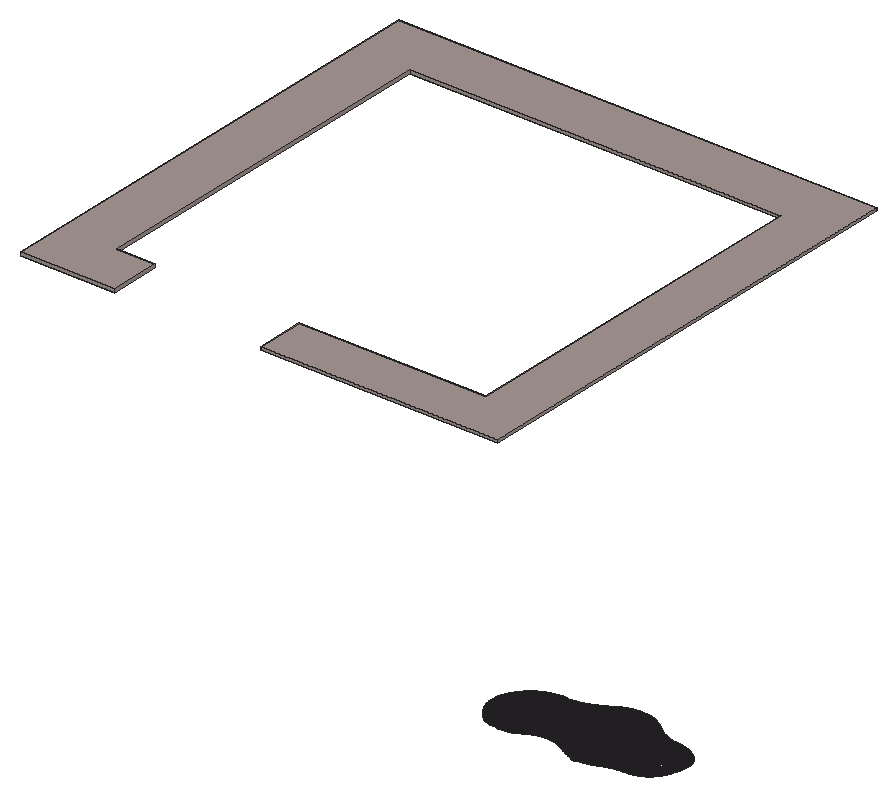
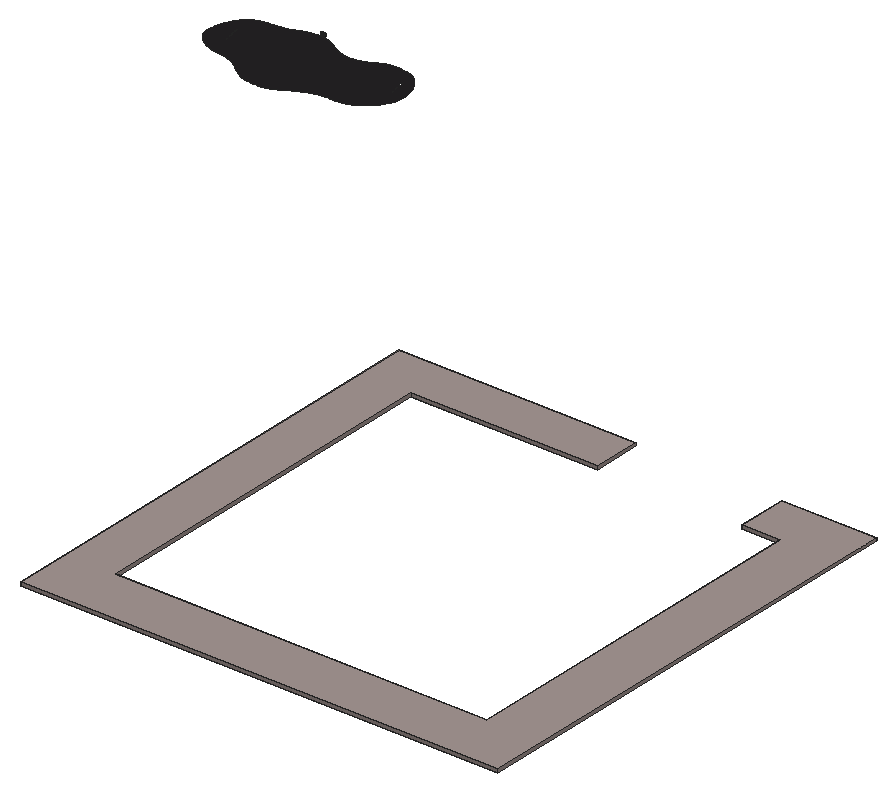
# SketchUp Ruby script. Lengths in inches.
U = 1.inch
M = Sketchup.active_model
def pt(a) = Geom::Point3d.new(a.map { |v| v * U })
def face(e, loops, mat)
  f = e.add_face(loops[0].map { |a| pt(a) })
  loops[1..].each { |l| e.add_face(l.map { |a| pt(a) }).erase! }
  f.material = f.back_material = mat if mat
  f
end
# faces: each face lists its corners as indices into pts; further lists are holes
def faces(e, pts, list, mat = nil) = list.each { |f| face(e, (f[0].is_a?(Array) ? f : [f]).map { |l| l.map { |i| pts[i] } }, mat) }
# xy, xz, yz: faces in a plane at the given z, y or x. An outline is a flat list of corners, or four numbers for a rectangle; further outlines are holes
def ring(l) = l.size == 4 ? [[l[0], l[1]], [l[2], l[1]], [l[2], l[3]], [l[0], l[3]]] : l.each_slice(2).to_a
def flat(e, list, mat, &to3) = list.each { |f| face(e, (f[0].is_a?(Array) ? f : [f]).map { |l| ring(l).map { |u, v| to3.(u, v) } }, mat) }
def xy(e, z, list, mat = nil) = flat(e, list, mat) { |x, y| [x, y, z] }
def xz(e, y, list, mat = nil) = flat(e, list, mat) { |x, z| [x, y, z] }
def yz(e, x, list, mat = nil) = flat(e, list, mat) { |y, z| [x, y, z] }
def lines(e, pts, list) = list.each { |a, b| e.add_line(pt(pts[a]), pt(pts[b])) }
# prism: a flat outline (further loops are holes) pulled along v
def prism(e, loops, v, mat = nil)
  f = face(e, loops, mat); d = Geom::Vector3d.new(v.map { |x| x * U })
  f.pushpull(f.normal.samedirection?(d) ? d.length : -d.length)
end
def box(e, o, s, mat = nil) = prism(e, [[o, [o[0] + s[0], o[1], o[2]], [o[0] + s[0], o[1] + s[1], o[2]], [o[0], o[1] + s[1], o[2]]]], [0, 0, s[2]], mat)
def at(x, y, z, deg = 0) = Geom::Transformation.translation(pt([x, y, z])) * Geom::Transformation.rotation(ORIGIN, Z_AXIS, deg.degrees)
def axes(o, x, y, z) = Geom::Transformation.new([*x, 0, *y, 0, *z, 0, *pt(o).to_a, 1])
def part(name) = M.definitions.add(name)
# library, detail: a bought-in or finely detailed component or shape, given as its bounding box
def library(name, o, s) = part(name).tap { |d| box(d.entities, o, s) }
def detail(e, o, s) = box(e.add_group.entities, o, s)
def put(e, d, t, mat = nil) = e.add_instance(d, t).tap { |i| i.material = mat if mat }
def group(e, t, mat = nil) = e.add_group.tap { |g| g.transformation = t; g.material = mat if mat }.entities
root = M.entities
M.materials.add("Marble_06_1K").color = [165, 150, 147]
M.materials.add("Marble_07_1K").color = [36, 34, 36]
xy(root,18,[[[347.35,773.18,347.67,773.18,347.88,773.19,347.99,773.19,348.1,773.2,348.2,773.21,348.31,773.21,348.42,773.22,348.52,773.23,348.73,773.25,348.83,773.26,349.01,773.28,349.1,773.3,349.19,773.31,349.43,773.34,349.51,773.36,349.59,773.37,349.66,773.38,349.74,773.4,349.81,773.41,349.89,773.43,349.97,773.44,350.04,773.46,350.12,773.47,350.19,773.49,350.27,773.5,350.34,773.52,350.42,773.54,350.49,773.55,350.57,773.57,350.64,773.59,350.72,773.61,350.79,773.625,350.87,773.64,350.94,773.66,351.02,773.68,351.09,773.7,351.17,773.72,351.24,773.74,351.32,773.76,351.39,773.78,351.46,773.81,351.54,773.83,351.68,773.87,351.76,773.89,351.83,773.92,351.91,773.94,351.98,773.96,352.05,773.99,352.125,774.01,352.2,774.04,352.27,774.0625,352.34,774.09,352.42,774.11,352.49,774.14,352.5625,774.17,352.63,774.19,352.71,774.22,352.78,774.25,352.85,774.27,352.99,774.33,353.07,774.36,353.42,774.51,353.5,774.54,353.64,774.6,353.72,774.63,353.8,774.67,353.96,774.73,354.04,774.77,354.13,774.8,354.21,774.84,354.39,774.91,354.48,774.94,354.57,774.98,354.65,775.01,354.83,775.07,354.92,775.11,355.19,775.2,355.28,775.22,355.55,775.31,355.64,775.33,355.73,775.36,355.82,775.38,355.92,775.41,356.1,775.45,356.19,775.48,356.28,775.5,356.47,775.54,356.65,775.58,356.75,775.59,356.84,775.61,356.94,775.63,357.03,775.65,357.13,775.66,357.35,775.7,357.46,775.71,357.58,775.73,357.71,775.74,357.86,775.76,358.02,775.78,358.2,775.79,358.4,775.81,358.64,775.82,358.9,775.84,359.2,775.84,359.53,775.85,359.87,775.87,360.59,775.93,360.96,775.97,361.31,776.01,361.66,776.06,361.99,776.11,362.3,776.18,362.6,776.24,362.89,776.32,363.16,776.39,363.43,776.48,363.69,776.57,363.95,776.67,364.2,776.77,364.45,776.89,364.7,777,364.94,777.125,365.18,777.26,365.42,777.39,365.65,777.53,366.11,777.83,366.33,777.99,366.55,778.16,366.76,778.33,366.97,778.51,367.17,778.7,367.55,779.1,367.91,779.54,368.23,780,368.39,780.24,368.53,780.49,368.68,780.74,368.82,780.99,369.08,781.51,369.32,782.03,369.43,782.3,369.54,782.5625,369.65,782.83,369.75,783.1,369.93,783.65,370.01,783.93,370.09,784.2,370.17,784.48,370.23,784.76,370.3,785.04,370.36,785.33,370.46,785.89,370.54,786.43,370.57,786.68,370.6,786.91,370.625,787.12,370.64,787.31,370.66,787.47,370.67,787.6,370.68,787.72,370.69,787.8125,370.6875,787.89,370.6875,788.08,370.68,788.14,370.68,788.26,370.67,788.32,370.67,788.38,370.66,788.4375,370.66,788.49,370.65,788.55,370.65,788.61,370.62,788.79,370.61,788.84,370.58,789.02,370.57,789.07,370.56,789.13,370.54,789.1875,370.53,789.25,370.51,789.3,370.5,789.36,370.48,789.42,370.47,789.47,370.45,789.53,370.44,789.59,370.42,789.64,370.4,789.7,370.38,789.75,370.36,789.81,370.34,789.86,370.32,789.92,370.3,789.97,370.28,790.03,370.26,790.08,370.23,790.14,370.21,790.19,370.1875,790.25,370.16,790.3,370.14,790.35,370.11,790.41,370.09,790.46,370.06,790.51,370.03,790.5625,370.01,790.61,369.98,790.67,369.77,791.02,369.73,791.07,369.67,791.17,369.63,791.21,369.57,791.31,369.53,791.36,369.49,791.4,369.46,791.45,369.42,791.49,369.38,791.54,369.35,791.59,369.27,791.67,369.23,791.72,369.19,791.76,369.15,791.81,368.99,791.97,368.95,792.02,368.91,792.06,368.86,792.1,368.78,792.18,368.73,792.21,368.6875,792.25,368.64,792.29,368.6,792.33,368.55,792.37,368.46,792.4375,368.42,792.47,368.375,792.51,368.33,792.54,368.29,792.58,368.17,792.67,368.13,792.69,368.1,792.72,368.07,792.74,368.05,792.76,368.03,792.77,368.01,792.79,367.99,792.8,367.98,792.8125,367.96,792.82,367.95,792.83,367.9375,792.84,367.93,792.85,367.92,792.86,367.9,792.86,367.89,792.875,367.87,792.89,367.78,792.95,367.74,792.98,367.69,793.01,367.64,793.05,367.58,793.08,367.52,793.125,367.45,793.17,367.39,793.21,367.32,793.25,367.25,793.3,367.11,793.38,367.05,793.42,366.42,793.78,366.35,793.8125,366.27,793.85,366.2,793.89,366.13,793.92,366.06,793.96,365.99,793.99,365.91,794.03,365.77,794.09,365.69,794.125,365.62,794.16,365.55,794.19,365.47,794.22,365.33,794.28,365.25,794.3125,365.18,794.34,365.1,794.37,365.03,794.4,364.95,794.43,364.875,794.46,364.8,794.48,364.72,794.51,364.65,794.54,364.57,794.5625,364.5,794.59,364.42,794.61,364.34,794.64,364.27,794.66,364.19,794.68,364.11,794.71,364.04,794.73,363.8,794.79,363.73,794.8125,363.65,794.83,363.41,794.89,363.34,794.91,363.26,794.93,363.18,794.94,363.1,794.96,363.02,794.97,362.94,794.99,362.86,795,362.79,795.02,362.71,795.03,362.63,795.05,362.39,795.08,362.31,795.1,362.15,795.12,362.07,795.125,361.99,795.14,361.91,795.14,361.67,795.17,361.58,795.18,361.5,795.18,361.41,795.19,361.3125,795.2,361.21,795.21,361.11,795.22,360.99,795.23,360.88,795.24,360.76,795.25,360.64,795.27,360.52,795.28,360.39,795.3,360.27,795.3125,360.14,795.33,360.02,795.35,359.89,795.37,359.77,795.39,359.64,795.42,359.52,795.44,359.39,795.47,359.27,795.49,359.15,795.52,359.02,795.55,358.66,795.64,358.54,795.68,358.41,795.71,357.93,795.87,357.8125,795.91,357.69,795.95,357.58,796,357.46,796.04,357.22,796.14,357.11,796.18,356.99,796.23,356.875,796.29,356.76,796.34,356.64,796.39,356.53,796.45,356.42,796.5,356.3,796.56,355.64,796.92,355.53,796.99,355.42,797.05,355.3125,797.12,355.21,797.19,355.1,797.26,355,797.33,354.89,797.4,354.79,797.47,354.69,797.55,354.58,797.62,354.48,797.69,354.38,797.77,354.02,798.05,353.94,798.11,353.87,798.17,353.81,798.22,353.74,798.27,353.68,798.32,353.63,798.37,353.57,798.41,353.52,798.45,353.47,798.5,353.32,798.62,353.26,798.66,353.06,798.82,353,798.86,352.9,798.94,352.84,798.98,352.79,799.02,352.74,799.0625,352.68,799.1,352.58,799.18,352.52,799.22,352.42,799.3,352.36,799.34,352.31,799.375,352.25,799.41,352.15,799.49,352.09,799.52,352.04,799.5625,351.98,799.6,351.93,799.64,351.87,799.67,351.82,799.71,351.76,799.75,351.71,799.78,351.65,799.82,351.59,799.85,351.54,799.89,351.48,799.93,351.43,799.96,351.37,800,351.31,800.03,351.26,800.07,351.2,800.1,351.15,800.14,351.09,800.17,351.03,800.21,350.98,800.24,350.92,800.27,350.86,800.31,350.8,800.34,350.75,800.375,350.69,800.41,350.63,800.44,350.58,800.47,350.52,800.51,350.34,800.6,350.29,800.63,350.23,800.67,350.17,800.7,350.12,800.73,350.07,800.75,350.02,800.78,349.97,800.8,349.93,800.83,349.85,800.87,349.8125,800.89,349.78,800.91,349.74,800.92,349.71,800.9375,349.68,800.95,349.64,800.97,349.61,800.99,349.58,801,349.55,801.02,349.51,801.03,349.48,801.05,349.45,801.0625,349.41,801.08,349.38,801.09,349.35,801.11,349.3125,801.12,349.28,801.14,349.25,801.15,349.21,801.16,349.18,801.18,349.15,801.19,349.11,801.2,349.08,801.22,349.04,801.23,349.01,801.24,348.98,801.26,348.94,801.27,348.91,801.28,348.875,801.3,348.84,801.31,348.81,801.32,348.77,801.33,348.74,801.34,348.7,801.36,348.67,801.37,348.63,801.38,348.6,801.39,348.56,801.4,348.5,801.42,348.46,801.44,348.43,801.45,348.39,801.46,348.36,801.47,348.32,801.48,348.29,801.49,348.25,801.5,348.22,801.51,348.18,801.52,348.15,801.53,348.11,801.54,348.08,801.55,348.04,801.55,348.01,801.5625,347.97,801.57,347.94,801.58,347.86,801.6,347.83,801.61,347.79,801.61,347.76,801.62,347.72,801.63,347.6875,801.64,347.65,801.65,347.62,801.65,347.54,801.67,347.51,801.67,347.47,801.68,347.4375,801.6875,347.4,801.69,347.37,801.7,347.33,801.71,347.29,801.71,347.26,801.72,347.22,801.72,347.1875,801.73,347.15,801.74,347.11,801.74,347.08,801.75,347.04,801.75,347.01,801.76,346.97,801.76,346.93,801.77,346.86,801.77,346.2,801.84,346.0625,801.85,345.91,801.86,345.59,801.88,345.23,801.9,345.04,801.91,344.85,801.91,344.66,801.92,344.1,801.92,343.93,801.91,343.77,801.91,343.61,801.9,343.47,801.89,343.21,801.86,343.09,801.84,342.97,801.83,342.85,801.81,342.74,801.79,342.51,801.75,342.4,801.72,342.29,801.7,342.17,801.68,342.0625,801.65,341.95,801.63,341.84,801.6,341.72,801.57,341.61,801.55,341.51,801.52,341.4,801.49,341.3,801.47,341.21,801.44,341.125,801.42,341.05,801.4,340.98,801.38,340.92,801.36,340.83,801.34,340.79,801.32,340.75,801.3125,340.72,801.3,340.6875,801.29,340.66,801.28,340.59,801.26,340.5625,801.25,340.53,801.24,340.44,801.21,340.4,801.19,340.25,801.14,340.22,801.125,340.18,801.11,340.09,801.08,340.06,801.0625,340.02,801.05,339.99,801.04,339.95,801.02,339.92,801.01,339.83,800.97,339.79,800.95,339.73,800.93,339.61,800.87,339.53,800.84,339.45,800.8,339.36,800.76,339.29,800.72,339.22,800.6875,339.16,800.66,339.11,800.63,338.95,800.55,338.89,800.51,338.85,800.49,338.82,800.48,338.76,800.44,338.73,800.43,338.71,800.41,338.68,800.39,338.62,800.36,338.59,800.34,338.5625,800.32,338.53,800.31,338.5,800.29,338.48,800.27,338.45,800.25,338.42,800.24,338.33,800.18,338.31,800.17,338.22,800.11,338.18,800.09,338.14,800.0625,338.1,800.03,338.04,800,337.97,799.96,337.89,799.91,337.8,799.85,337.6875,799.79,337.57,799.72,337.44,799.64,337.16,799.48,336.86,799.3,336.71,799.22,336.5625,799.13,336.41,799.05,336.25,798.96,336.09,798.875,335.92,798.78,335.74,798.69,335.36,798.49,335.14,798.38,334.91,798.27,334.64,798.14,334.34,797.99,334,797.83,333.61,797.65,333.17,797.45,332.96,797.34,332.76,797.25,332.59,797.17,332.44,797.1,332.31,797.04,332.1875,796.99,332.08,796.95,331.98,796.9,331.88,796.87,331.7,796.79,331.61,796.76,331.53,796.73,331.44,796.7,331.2,796.61,331.12,796.59,331.04,796.56,330.95,796.53,330.875,796.51,330.79,796.48,330.71,796.46,330.625,796.43,330.54,796.41,330.46,796.39,330.38,796.36,330.3,796.34,330.21,796.32,330.05,796.28,329.96,796.26,329.8,796.22,329.71,796.2,329.63,796.18,329.54,796.17,329.46,796.15,329.375,796.13,329.29,796.12,329.21,796.1,329.12,796.09,329.04,796.07,328.95,796.06,328.87,796.05,328.78,796.03,328.7,796.02,328.61,796.01,328.53,796,328.44,795.99,328.36,795.98,328.27,795.97,328.1875,795.96,328.1,795.95,328.02,795.94,327.93,795.9375,327.84,795.93,327.76,795.92,327.67,795.92,327.59,795.91,327.5,795.91,327.42,795.9,327.24,795.9,327.16,795.89,326.39,795.89,326.3,795.9,326.13,795.9,326.04,795.91,325.96,795.91,325.87,795.92,325.79,795.92,325.7,795.93,325.61,795.9375,325.52,795.94,325.42,795.95,325.19,795.95,325.07,795.96,324.93,795.96,324.79,795.95,324.63,795.95,324.47,795.94,324.3,795.94,324.13,795.92,323.79,795.9,323.61,795.88,323.4375,795.86,323.26,795.84,323.09,795.82,322.92,795.79,322.74,795.76,322.4,795.7,322.23,795.66,322.05,795.625,321.88,795.58,321.54,795.5,321.21,795.4,320.87,795.3,320.7,795.24,320.54,795.18,320.375,795.125,320.21,795.0625,320.05,795,319.88,794.93,319.72,794.86,319.5625,794.79,319.4,794.72,319.24,794.64,319.09,794.57,318.77,794.41,318.62,794.32,318.47,794.24,318.3125,794.15,318.16,794.0625,318.01,793.97,317.86,793.88,317.72,793.78,317.57,793.6875,317.43,793.59,317.28,793.49,317.14,793.38,317,793.28,316.86,793.17,316.72,793.0625,316.59,792.95,316.45,792.84,316.32,792.73,316.19,792.61,316.05,792.5,315.93,792.375,315.8,792.26,315.55,792.01,315.43,791.88,315.31,791.76,315.1875,791.63,315.07,791.5,314.95,791.37,314.84,791.23,314.73,791.1,314.4,790.68,314.3,790.54,314.19,790.4,314.09,790.26,313.89,789.96,313.79,789.8,313.68,789.64,313.58,789.46,313.36,789.1,313.25,788.9,313.13,788.7,313.02,788.5,312.92,788.3,312.8125,788.1,312.72,787.9,312.63,787.71,312.55,787.53,312.49,787.36,312.43,787.2,312.375,787.04,312.33,786.88,312.25,786.58,312.22,786.43,312.1875,786.29,312.16,786.14,312.1,785.84,312.08,785.6875,312.06,785.54,312.04,785.39,312.02,785.23,312.01,785.08,311.99,784.93,311.97,784.63,311.97,784.48,311.96,784.32,311.96,783.87,311.97,783.72,311.97,783.5625,311.98,783.41,312,783.11,312.02,782.96,312.03,782.81,312.07,782.51,312.09,782.35,312.12,782.2,312.14,782.05,312.17,781.91,312.2,781.76,312.24,781.61,312.27,781.46,312.31,781.3125,312.35,781.16,312.39,781.01,312.4375,780.85,312.49,780.6875,312.55,780.52,312.61,780.35,312.68,780.16,312.75,779.96,312.84,779.75,312.95,779.51,313.07,779.25,313.39,778.61,313.59,778.23,313.84,777.88,314.0625,777.58,314.26,777.3125,314.45,777.08,314.61,776.88,314.76,776.71,314.91,776.55,315.04,776.41,315.17,776.28,315.29,776.15,315.42,776.03,315.54,775.92,315.65,775.8125,315.77,775.71,315.89,775.61,316,775.51,316.12,775.41,316.36,775.23,316.49,775.14,316.61,775.05,316.74,774.96,317,774.8,317.28,774.64,317.43,774.57,317.59,774.49,317.76,774.42,317.94,774.35,318.14,774.27,318.36,774.2,318.6,774.125,318.86,774.05,319.13,773.98,319.42,773.91,319.72,773.84,320.34,773.72,321.3,773.6,321.62,773.58,322.26,773.56,322.58,773.56,322.91,773.57,323.23,773.59,323.55,773.62,323.86,773.65,324.17,773.6875,324.47,773.73,324.76,773.78,325.02,773.83,325.27,773.88,325.5,773.93,325.69,773.98,325.87,774.02,326.03,774.07,326.18,774.12,326.32,774.17,326.45,774.23,326.59,774.29,326.74,774.36,326.89,774.44,327.23,774.62,327.77,774.92,327.95,775.03,328.31,775.23,328.65,775.43,328.99,775.61,329.15,775.7,329.49,775.88,329.65,775.96,329.99,776.12,330.17,776.2,330.51,776.34,330.6875,776.41,330.86,776.47,331.04,776.54,331.22,776.6,331.39,776.65,331.57,776.71,331.75,776.76,331.93,776.8125,332.12,776.86,332.3,776.9,332.48,776.95,332.66,776.98,332.85,777.02,333.03,777.05,333.22,777.08,333.4,777.11,333.59,777.14,333.78,777.16,333.96,777.18,334.15,777.2,334.34,777.21,334.52,777.22,334.9,777.24,335.46,777.24,335.64,777.23,335.82,777.23,336,777.22,336.17,777.21,336.32,777.19,336.46,777.18,336.59,777.17,336.71,777.15,336.8,777.13,336.89,777.12,337.03,777.08,337.09,777.0625,337.15,777.04,337.2,777.02,337.25,777.01,337.31,776.99,337.41,776.95,337.47,776.93,337.57,776.89,337.68,776.85,337.78,776.81,337.84,776.79,337.89,776.76,337.99,776.72,338.05,776.7,338.2,776.64,338.26,776.62,338.31,776.59,338.41,776.55,338.47,776.53,338.52,776.51,338.57,776.48,338.62,776.46,338.67,776.4375,338.73,776.42,338.78,776.39,338.88,776.35,338.93,776.32,338.98,776.3,339.04,776.28,339.09,776.25,339.14,776.23,339.19,776.2,339.29,776.16,339.34,776.13,339.4,776.11,339.45,776.08,339.5,776.06,339.55,776.03,339.6,776.01,339.65,775.98,339.7,775.96,339.75,775.93,339.8,775.91,339.85,775.88,339.9,775.86,340,775.8,340.05,775.78,340.1,775.75,340.16,775.73,340.26,775.67,340.31,775.65,340.41,775.59,340.45,775.57,340.6,775.48,340.65,775.46,340.85,775.34,340.9,775.32,341.15,775.17,341.19,775.14,341.24,775.12,341.44,775,341.49,774.96,341.61,774.9,341.67,774.86,341.74,774.82,341.8125,774.78,341.89,774.73,341.97,774.68,342.33,774.48,342.43,774.43,342.52,774.38,342.62,774.34,342.71,774.29,342.81,774.24,342.9,774.2,343,774.15,343.3,774.03,343.39,773.99,343.79,773.83,343.89,773.8,343.99,773.76,344.1,773.73,344.2,773.7,344.3,773.66,344.5,773.6,344.61,773.57,344.71,773.55,344.8125,773.52,344.92,773.49,345.02,773.47,345.125,773.45,345.23,773.42,345.33,773.4,345.4375,773.38,345.54,773.36,345.65,773.34,345.75,773.32,345.86,773.31,345.97,773.29,346.07,773.28,346.18,773.26,346.28,773.25,346.5,773.23,346.6,773.22,346.71,773.21,346.82,773.21,346.92,773.2,347.03,773.19,347.14,773.19,347.24,773.1875],[365.49,782.54,365.4375,782.55,365.375,782.55,365.29,782.58,365.19,782.6,365.1,782.61,365.01,782.63,364.91,782.65,364.85,782.65,364.76,782.74,364.76,782.79,364.79,782.83,364.81,782.88,364.83,782.92,364.86,782.97,364.875,783.01,364.9,783.07,364.92,783.12,364.93,783.16,364.93,783.26,364.92,783.3,364.88,783.42,364.85,783.47,364.83,783.52,364.77,783.64,364.76,783.68,364.73,783.74,364.71,783.8,364.7,783.85,364.7,783.89,364.68,783.97,364.68,784.04,364.67,784.08,364.66,784.16,364.67,784.2,364.67,784.26,364.66,784.33,364.66,784.38,364.67,784.43,364.67,784.48,364.7,784.53,364.72,784.58,364.72,784.625,364.75,784.67,364.77,784.71,364.79,784.76,364.82,784.8125,364.84,784.86,364.85,784.9,364.87,784.95,364.88,785.01,364.83,785.11,364.8,785.16,364.78,785.2,364.74,785.24,364.65,785.39,364.62,785.4375,364.6,785.48,364.57,785.52,364.55,785.5625,364.52,785.61,364.49,785.66,364.45,785.71,364.43,785.77,364.375,785.88,364.36,785.92,364.33,785.99,364.3,786.04,364.3,786.14,364.29,786.21,364.3,786.28,364.3125,786.35,364.32,786.41,364.33,786.46,364.35,786.51,364.36,786.57,364.37,786.62,364.37,786.66,364.38,786.71,364.39,786.75,364.375,786.83,364.35,786.87,364.34,786.92,364.33,786.96,364.3,787,364.28,787.05,364.26,787.09,364.24,787.14,364.23,787.18,364.21,787.24,364.2,787.28,364.17,787.33,364.16,787.375,364.13,787.44,364.12,787.49,364.1,787.52,364.08,787.58,364.06,787.625,364.04,787.68,364.03,787.72,364.01,787.78,363.99,787.83,363.99,787.875,363.97,787.93,363.97,787.97,363.98,788.04,363.97,788.1,363.99,788.14,363.98,788.1875,363.99,788.24,363.99,788.3,364,788.36,364,788.41,363.98,788.51,363.99,788.55,363.97,788.6,363.96,788.64,363.96,788.6875,363.9375,788.73,363.93,788.77,363.91,788.81,363.9,788.85,363.89,788.9,363.88,788.9375,363.86,788.98,363.84,789.04,363.83,789.08,363.81,789.125,363.79,789.18,363.77,789.28,363.75,789.33,363.74,789.38,363.72,789.46,363.72,789.52,363.71,789.54,363.68,789.67,363.71,789.75,363.86,789.71,363.9,789.68,363.96,789.62,364,789.59,364.03,789.55,364.06,789.52,364.08,789.47,364.12,789.42,364.14,789.37,364.15,789.33,364.16,789.28,364.17,789.24,364.19,789.19,364.2,789.15,364.21,789.1,364.23,789.05,364.24,789.01,364.27,788.97,364.3,788.92,364.36,788.84,364.38,788.79,364.41,788.75,364.44,788.72,364.46,788.66,364.49,788.63,364.5,788.59,364.53,788.54,364.57,788.44,364.57,788.3,364.58,788.27,364.59,788.2,364.59,788.16,364.57,788.11,364.58,788.0625,364.56,788.02,364.54,787.98,364.53,787.93,364.52,787.87,364.53,787.83,364.52,787.78,364.52,787.73,364.51,787.69,364.52,787.64,364.52,787.6,364.53,787.56,364.55,787.46,364.58,787.42,364.59,787.38,364.61,787.34,364.66,787.29,364.6875,787.25,364.71,787.21,364.75,787.17,364.79,787.11,364.83,787.07,364.86,787.05,364.9,786.99,364.9375,786.95,364.97,786.92,365.01,786.87,365.05,786.83,365.08,786.78,365.1,786.74,365.13,786.6875,365.14,786.63,365.14,786.52,365.12,786.48,365.09,786.44,365.06,786.41,365.03,786.37,365.02,786.33,364.99,786.28,364.95,786.18,364.95,786.07,364.96,786.02,364.99,785.97,365.02,785.93,365.04,785.89,365.07,785.84,365.09,785.78,365.11,785.7,365.13,785.64,365.15,785.54,365.17,785.49,365.18,785.4375,365.19,785.39,365.2,785.35,365.22,785.29,365.23,785.24,365.23,785.09,365.22,785.03,365.22,784.97,365.2,784.92,365.21,784.88,365.21,784.83,365.19,784.79,365.2,784.74,365.18,784.64,365.21,784.59,365.23,784.55,365.26,784.5,365.32,784.41,365.35,784.38,365.39,784.33,365.43,784.26,365.47,784.22,365.49,784.18,365.52,784.14,365.56,784.07,365.59,784.03,365.61,783.98,365.63,783.92,365.64,783.875,365.65,783.81,365.65,783.76,365.64,783.7,365.55,783.55,365.47,783.39,365.44,783.34,365.42,783.28,365.4,783.24,365.38,783.1875,365.36,783.14,365.36,783.08,365.35,783.03,365.36,782.98,365.375,782.93,365.39,782.89,365.42,782.83,365.4375,782.78,365.45,782.75,365.5,782.67,365.51,782.62,365.54,782.54],[317.04,778.3125,316.99,778.32,316.93,778.33,316.75,778.37,316.65,778.38,316.57,778.4,316.47,778.42,316.41,778.43,316.35,778.48,316.3125,778.52,316.32,778.5625,316.34,778.61,316.36,778.65,316.39,778.7,316.43,778.78,316.46,778.85,316.48,778.89,316.49,778.9375,316.48,778.99,316.49,779.03,316.47,779.08,316.46,779.13,316.4,779.25,316.39,779.3,316.36,779.33,316.33,779.41,316.3125,779.45,316.29,779.52,316.27,779.58,316.26,779.62,316.26,779.66,316.23,779.75,316.24,779.8125,316.23,779.86,316.22,779.93,316.23,779.98,316.22,780.03,316.21,780.1,316.21,780.15,316.22,780.21,316.23,780.26,316.25,780.31,316.27,780.35,316.28,780.4,316.3,780.44,316.32,780.49,316.35,780.53,316.375,780.59,316.39,780.63,316.41,780.68,316.42,780.72,316.44,780.79,316.42,780.83,316.36,780.93,316.33,780.97,316.3,781.02,316.26,781.06,316.23,781.11,316.21,781.17,316.18,781.21,316.16,781.26,316.125,781.3,316.1,781.34,316.07,781.39,316.04,781.4375,316.01,781.49,315.99,781.55,315.93,781.65,315.91,781.7,315.88,781.76,315.86,781.8125,315.86,781.87,315.85,781.92,315.84,781.98,315.86,782.06,315.87,782.125,315.88,782.1875,315.88,782.23,315.9,782.29,315.91,782.35,315.93,782.39,315.93,782.4375,315.9375,782.48,315.94,782.52,315.93,782.6,315.91,782.65,315.9,782.6875,315.88,782.73,315.86,782.78,315.83,782.82,315.82,782.87,315.8,782.91,315.76,783.01,315.75,783.05,315.71,783.15,315.68,783.21,315.68,783.26,315.66,783.29,315.64,783.35,315.61,783.4,315.6,783.46,315.59,783.5,315.55,783.6,315.53,783.7,315.53,783.75,315.54,783.81,315.53,783.87,315.54,783.91,315.54,784.02,315.55,784.07,315.55,784.23,315.54,784.29,315.54,784.33,315.52,784.37,315.52,784.41,315.51,784.46,315.49,784.51,315.48,784.55,315.46,784.59,315.46,784.63,315.45,784.67,315.4375,784.71,315.41,784.76,315.4,784.8125,315.39,784.86,315.36,784.9,315.35,784.96,315.33,785.01,315.32,785.05,315.31,785.11,315.29,785.15,315.29,785.19,315.28,785.23,315.28,785.29,315.27,785.32,315.24,785.44,315.26,785.53,315.42,785.48,315.45,785.45,315.49,785.42,315.62,785.29,315.64,785.24,315.67,785.19,315.69,785.15,315.7,785.1,315.72,785.06,315.73,785.02,315.75,784.97,315.75,784.92,315.76,784.875,315.78,784.83,315.8,784.79,315.83,784.75,315.85,784.7,315.91,784.62,315.9375,784.57,315.97,784.53,316,784.49,316.02,784.4375,316.05,784.4,316.06,784.36,316.08,784.31,316.1,784.27,316.12,784.22,316.125,784.17,316.13,784.13,316.13,784.08,316.14,784.04,316.14,783.93,316.125,783.89,316.13,783.84,316.12,783.79,316.1,783.75,316.09,783.71,316.08,783.65,316.08,783.51,316.07,783.46,316.07,783.42,316.09,783.33,316.1,783.29,316.1,783.24,316.13,783.19,316.15,783.15,316.21,783.06,316.25,783.02,316.27,782.99,316.3,782.94,316.35,782.88,316.41,782.82,316.45,782.76,316.49,782.73,316.52,782.7,316.57,782.64,316.6,782.61,316.66,782.51,316.7,782.41,316.7,782.3,316.67,782.26,316.65,782.22,316.61,782.18,316.57,782.1,316.51,781.95,316.5,781.9,316.51,781.85,316.52,781.79,316.55,781.74,316.58,781.7,316.65,781.56,316.65,781.51,316.67,781.47,316.69,781.41,316.7,781.36,316.71,781.32,316.73,781.26,316.74,781.21,316.75,781.17,316.76,781.125,316.78,781.07,316.78,781.02,316.79,780.98,316.79,780.86,316.78,780.8,316.78,780.74,316.76,780.7,316.76,780.6,316.75,780.56,316.75,780.51,316.74,780.47,316.73,780.41,316.79,780.33,316.82,780.28,316.84,780.24,316.875,780.1875,316.91,780.16,316.94,780.1,316.99,780.03,317.05,779.95,317.07,779.92,317.11,779.84,317.15,779.8,317.16,779.76,317.18,779.69,317.19,779.65,317.21,779.58,317.2,779.53,317.19,779.47,317.17,779.42,317.08,779.27,317.06,779.22,317.02,779.16,317,779.11,316.97,779.06,316.93,778.96,316.92,778.91,316.92,778.86,316.91,778.81,316.93,778.71,316.95,778.66,316.97,778.6,316.99,778.56,317,778.52,317.05,778.44,317.07,778.39,317.09,778.3125]]],"Marble_07_1K")
xz(root,772.58,[[347.23,18,347.34,19]],"Marble_07_1K")
xz(root,772.59,[[347,18,347.12,19]],"Marble_07_1K")
xz(root,772.6,[[346.78,18,346.89,19]],"Marble_07_1K")
p = [[346.22,772.65,18],[346.33,772.64,18],[346.33,772.64,19],[346.22,772.65,19],[346.44,772.63,18],[346.44,772.63,19],
  [346.55,772.62,18],[346.55,772.62,19],[346.67,772.61,18],[346.67,772.61,19],[346.78,772.6,18],[346.78,772.6,19],
  [346.89,772.6,18],[347,772.59,18],[347,772.59,19],[346.89,772.6,19],[347.12,772.59,18],[347.23,772.58,18],
  [347.23,772.58,19],[347.12,772.59,19],[345.77,772.71,18],[345.88,772.69,18],[345.88,772.69,19],[345.77,772.71,19],
  [345.99,772.68,18],[345.99,772.68,19],[346.1,772.67,18],[346.1,772.67,19]]
faces(root,p,[[0,1,2,3],[1,4,5,2],[4,6,7,5],[6,8,9,7],[8,10,11,9],[12,13,14,15],[16,17,18,19],[20,21,22,23],
  [21,24,25,22],[24,26,27,25],[26,0,3,27]],"Marble_07_1K")
g1 = group(root,at(82.69,885.05,19),"Marble_06_1K")
prism(g1,[[[29.74,16.05,-1],[29.74,0.21,-1],[0,0.21,-1],[0,148.78,-1],[150.14,148.78,-1],[150.14,0,-1],[75.74,0,-1],[75.74,15.05,-1],[134.3,15.05,-1],[134.3,131.04,-1],[17.8,131.04,-1],[17.8,16.05,-1]]],[0,0,1])
